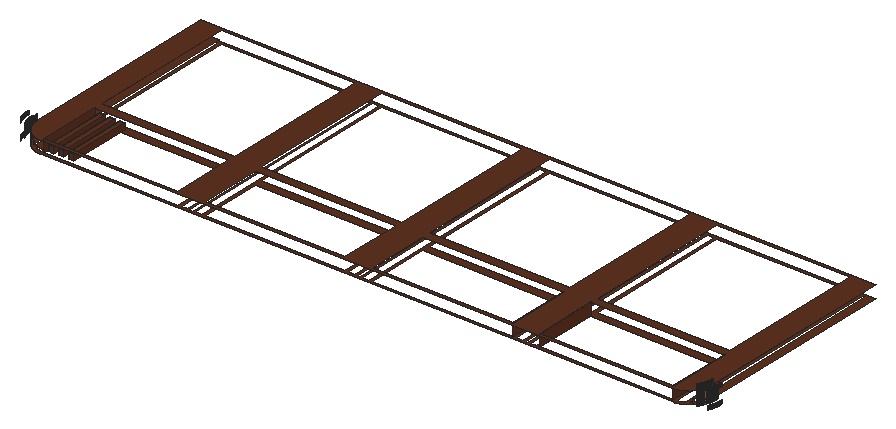
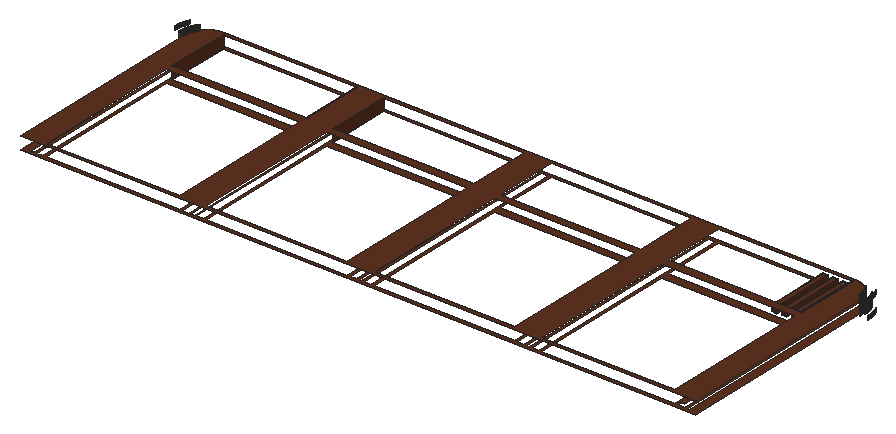
# SketchUp Ruby script. Lengths in inches.
U = 1.inch
M = Sketchup.active_model
def pt(a) = Geom::Point3d.new(a.map { |v| v * U })
def face(e, loops, mat)
  f = e.add_face(loops[0].map { |a| pt(a) })
  loops[1..].each { |l| e.add_face(l.map { |a| pt(a) }).erase! }
  f.material = f.back_material = mat if mat
  f
end
# faces: each face lists its corners as indices into pts; further lists are holes
def faces(e, pts, list, mat = nil) = list.each { |f| face(e, (f[0].is_a?(Array) ? f : [f]).map { |l| l.map { |i| pts[i] } }, mat) }
# xy, xz, yz: faces in a plane at the given z, y or x. An outline is a flat list of corners, or four numbers for a rectangle; further outlines are holes
def ring(l) = l.size == 4 ? [[l[0], l[1]], [l[2], l[1]], [l[2], l[3]], [l[0], l[3]]] : l.each_slice(2).to_a
def flat(e, list, mat, &to3) = list.each { |f| face(e, (f[0].is_a?(Array) ? f : [f]).map { |l| ring(l).map { |u, v| to3.(u, v) } }, mat) }
def xy(e, z, list, mat = nil) = flat(e, list, mat) { |x, y| [x, y, z] }
def xz(e, y, list, mat = nil) = flat(e, list, mat) { |x, z| [x, y, z] }
def yz(e, x, list, mat = nil) = flat(e, list, mat) { |y, z| [x, y, z] }
def lines(e, pts, list) = list.each { |a, b| e.add_line(pt(pts[a]), pt(pts[b])) }
# prism: a flat outline (further loops are holes) pulled along v
def prism(e, loops, v, mat = nil)
  f = face(e, loops, mat); d = Geom::Vector3d.new(v.map { |x| x * U })
  f.pushpull(f.normal.samedirection?(d) ? d.length : -d.length)
end
def box(e, o, s, mat = nil) = prism(e, [[o, [o[0] + s[0], o[1], o[2]], [o[0] + s[0], o[1] + s[1], o[2]], [o[0], o[1] + s[1], o[2]]]], [0, 0, s[2]], mat)
def at(x, y, z, deg = 0) = Geom::Transformation.translation(pt([x, y, z])) * Geom::Transformation.rotation(ORIGIN, Z_AXIS, deg.degrees)
def axes(o, x, y, z) = Geom::Transformation.new([*x, 0, *y, 0, *z, 0, *pt(o).to_a, 1])
def part(name) = M.definitions.add(name)
# library, detail: a bought-in or finely detailed component or shape, given as its bounding box
def library(name, o, s) = part(name).tap { |d| box(d.entities, o, s) }
def detail(e, o, s) = box(e.add_group.entities, o, s)
def put(e, d, t, mat = nil) = e.add_instance(d, t).tap { |i| i.material = mat if mat }
def group(e, t, mat = nil) = e.add_group.tap { |g| g.transformation = t; g.material = mat if mat }.entities
root = M.entities
M.materials.add("1799 AP 8574 BURNISHED CARAMEL").color = [140, 96, 69]
M.materials.add("1816 AP K197 Dark Kaapi-N").color = [79, 50, 27]
M.materials.add("[Wood Cherry Original]1").color = [93, 50, 33]
c1 = part("3")
box(c1.entities,[0,0,0],[3,2,36])
xy(root,391,[[[65.66,83,64.81,83.05,64.13,83.13,63.97,83.16,63.8,83.1875,63.63,83.22,63.46,83.25,63.3,83.28,63.13,83.32,62.97,83.36,62.8,83.4,62.64,83.44,62.47,83.49,62.31,83.54,62.14,83.58,61.98,83.64,61.82,83.69,61.66,83.75,61.5,83.8,61.34,83.86,61.18,83.93,61.03,83.99,60.87,84.06,60.71,84.125,60.56,84.19,60.4,84.27,60.25,84.34,59.65,84.66,59.52,84.73,59.5,84.74,59.35,84.83,59.21,84.92,59.0625,85.01,58.92,85.1,58.78,85.19,58.64,85.29,58.5,85.38,58.22,85.58,58.09,85.6875,57.95,85.79,57.82,85.9,57.6875,86.01,57.56,86.11,57.52,86.15,57.43,86.23,57.3,86.34,57.18,86.45,57.05,86.57,56.93,86.6875,56.81,86.81,56.6875,86.93,56.57,87.05,56.45,87.18,56.34,87.3,56.23,87.43,56.11,87.56,56.01,87.6875,55.9,87.82,55.79,87.95,55.6875,88.09,55.58,88.22,55.38,88.5,55.29,88.64,55.19,88.78,55.1,88.92,55.01,89.0625,54.92,89.21,54.83,89.35,54.74,89.5,54.34,90.25,54.27,90.4,54.19,90.56,54.125,90.71,54.06,90.87,53.99,91.03,53.93,91.18,53.86,91.34,53.8,91.5,53.75,91.66,53.69,91.82,53.64,91.98,53.58,92.14,53.54,92.31,53.49,92.47,53.44,92.64,53.4,92.8,53.36,92.97,53.32,93.13,53.28,93.3,53.25,93.46,53.22,93.63,53.1875,93.8,53.16,93.97,53.13,94.13,53.05,94.81,53,95.66,53,211,433,211,433,95.66,432.95,94.81,432.87,94.13,432.84,93.97,432.8125,93.8,432.78,93.63,432.75,93.46,432.72,93.3,432.68,93.13,432.64,92.97,432.6,92.8,432.56,92.64,432.51,92.47,432.46,92.31,432.42,92.14,432.36,91.98,432.31,91.82,432.25,91.66,432.2,91.5,432.14,91.34,432.07,91.18,432.01,91.03,431.94,90.87,431.875,90.71,431.81,90.56,431.73,90.4,431.66,90.25,431.26,89.5,431.17,89.35,431.08,89.21,430.99,89.0625,430.9,88.92,430.81,88.78,430.71,88.64,430.62,88.5,430.42,88.22,430.3125,88.09,430.21,87.95,430.1,87.82,429.99,87.6875,429.89,87.56,429.77,87.43,429.66,87.3,429.55,87.18,429.43,87.05,429.3125,86.93,429.19,86.81,429.07,86.6875,428.95,86.57,428.82,86.45,428.7,86.34,428.57,86.23,428.48,86.15,428.44,86.11,428.3125,86.01,428.18,85.9,428.05,85.79,427.91,85.6875,427.78,85.58,427.5,85.38,427.36,85.29,427.22,85.19,427.08,85.1,426.9375,85.01,426.79,84.92,426.65,84.83,426.5,84.74,426.48,84.73,426.35,84.66,425.75,84.34,425.6,84.27,425.44,84.19,425.29,84.125,425.13,84.06,424.97,83.99,424.82,83.93,424.66,83.86,424.5,83.8,424.34,83.75,424.18,83.69,424.02,83.64,423.86,83.58,423.69,83.54,423.53,83.49,423.36,83.44,423.2,83.4,423.03,83.36,422.87,83.32,422.7,83.28,422.54,83.25,422.37,83.22,422.2,83.1875,422.03,83.16,421.87,83.13,421.19,83.05,420.34,83],[156.25,124.5,235.5,209.5],[250.5,124.5,329.75,209.5],[66.02,124.5,141.25,209.5],[344.75,124.5,419.98,209.5],[250.5,84.5,329.75,120.5],[156.25,84.5,235.5,120.5],[344.75,84.5,419.98,120.5],[66.02,84.5,141.25,120.5],[142.75,84.5,146.75,209.5],[150.75,84.5,154.75,209.5],[245,84.5,249,209.5],[237,84.5,241,209.5],[339.25,84.5,343.25,209.5],[331.25,84.5,335.25,209.5],[421.48,84.6,421.5,84.6,421.8,84.64,422.1,84.69,422.24,84.72,422.54,84.78,422.83,84.85,423.12,84.93,423.7,85.11,423.98,85.21,424.4,85.375,424.68,85.49,424.95,85.62,425.09,85.6875,425.35,85.82,425.48,85.89,425.48,209.5,421.48,209.5],[64.52,84.61,64.52,209.5,60.52,209.5,60.52,85.9,60.99,85.66,61.47,85.43,61.96,85.24,62.46,85.0625,62.97,84.91,63.48,84.78,64,84.68],[147.75,84.5,149.75,209.5],[242,84.5,244,209.5],[336.25,84.5,338.25,209.5],[426.48,86.5,426.51,86.52,426.64,86.61,427.12,86.97,427.35,87.16,427.47,87.26,427.69,87.45,427.81,87.56,428.02,87.76,428.34,88.08,428.48,88.23,428.48,209.5,426.48,209.5],[59.52,86.5,59.52,209.5,57.52,209.5,57.52,88.23,57.66,88.08,58.08,87.66,58.19,87.56,58.42,87.35,58.88,86.97,59.24,86.7,59.49,86.52]]],"[Wood Cherry Original]1")
xy(root,392.75,[[65.85,84.5,66.02,84.5,65.45,84.52,64.875,84.5625,64.52,84.61,64.3,84.64,63.74,84.74,63.18,84.87,62.625,85.02,62.08,85.2,61.54,85.41,61.02,85.65,60.52,85.9,60.52,209.5,64.52,209.5,64.52,84.6,64.8,84.5625,65.1,84.54,65.55,84.51]],"[Wood Cherry Original]1")
xy(root,398,[[[65.66,83,420.34,83,421.19,83.05,421.87,83.13,422.03,83.16,422.2,83.1875,422.37,83.22,422.54,83.25,422.7,83.28,422.87,83.32,423.03,83.36,423.2,83.4,423.36,83.44,423.53,83.49,423.69,83.54,423.86,83.58,424.02,83.64,424.18,83.69,424.34,83.75,424.5,83.8,424.66,83.86,424.82,83.93,424.97,83.99,425.13,84.06,425.29,84.125,425.44,84.19,425.6,84.27,425.75,84.34,426.5,84.74,426.65,84.83,426.79,84.92,426.9375,85.01,427.08,85.1,427.22,85.19,427.36,85.29,427.5,85.38,427.78,85.58,427.91,85.6875,428.05,85.79,428.18,85.9,428.3125,86.01,428.44,86.11,428.57,86.23,428.7,86.34,428.82,86.45,428.95,86.57,429.07,86.6875,429.19,86.81,429.3125,86.93,429.43,87.05,429.55,87.18,429.66,87.3,429.77,87.43,429.89,87.56,429.99,87.6875,430.1,87.82,430.21,87.95,430.3125,88.09,430.42,88.22,430.62,88.5,430.71,88.64,430.81,88.78,430.9,88.92,430.99,89.0625,431.08,89.21,431.17,89.35,431.26,89.5,431.66,90.25,431.73,90.4,431.81,90.56,431.875,90.71,431.94,90.87,432.01,91.03,432.07,91.18,432.14,91.34,432.2,91.5,432.25,91.66,432.31,91.82,432.36,91.98,432.42,92.14,432.46,92.31,432.51,92.47,432.56,92.64,432.6,92.8,432.64,92.97,432.68,93.13,432.72,93.3,432.75,93.46,432.78,93.63,432.8125,93.8,432.84,93.97,432.87,94.13,432.95,94.81,433,95.66,433,211,53,211,53,95.66,53.05,94.81,53.13,94.13,53.16,93.97,53.1875,93.8,53.22,93.63,53.25,93.46,53.28,93.3,53.32,93.13,53.36,92.97,53.4,92.8,53.44,92.64,53.49,92.47,53.54,92.31,53.58,92.14,53.64,91.98,53.69,91.82,53.75,91.66,53.8,91.5,53.86,91.34,53.93,91.18,53.99,91.03,54.06,90.87,54.125,90.71,54.19,90.56,54.27,90.4,54.34,90.25,54.74,89.5,54.83,89.35,54.92,89.21,55.01,89.0625,55.1,88.92,55.19,88.78,55.29,88.64,55.38,88.5,55.58,88.22,55.6875,88.09,55.79,87.95,55.9,87.82,56.01,87.6875,56.11,87.56,56.23,87.43,56.34,87.3,56.45,87.18,56.57,87.05,56.6875,86.93,56.81,86.81,56.93,86.6875,57.05,86.57,57.18,86.45,57.3,86.34,57.43,86.23,57.56,86.11,57.6875,86.01,57.82,85.9,57.95,85.79,58.09,85.6875,58.22,85.58,58.5,85.38,58.64,85.29,58.78,85.19,58.92,85.1,59.0625,85.01,59.21,84.92,59.35,84.83,59.5,84.74,60.25,84.34,60.4,84.27,60.56,84.19,60.71,84.125,60.87,84.06,61.03,83.99,61.18,83.93,61.34,83.86,61.5,83.8,61.66,83.75,61.82,83.69,61.98,83.64,62.14,83.58,62.31,83.54,62.47,83.49,62.64,83.44,62.8,83.4,62.97,83.36,63.13,83.32,63.3,83.28,63.46,83.25,63.63,83.22,63.8,83.1875,63.97,83.16,64.13,83.13,64.81,83.05],[344.75,84.5,344.75,209.5,419.98,209.5,419.98,124.5,344.75,124.5,344.75,120.5,419.98,120.5,419.98,84.5],[156.25,124.5,235.5,209.5],[250.5,124.5,329.75,209.5],[66.02,124.5,141.25,209.5],[250.5,84.5,329.75,120.5],[156.25,84.5,235.5,120.5],[66.02,84.5,141.25,120.5]]],"[Wood Cherry Original]1")
yz(root,48,[[95.76,390,96,392],[95.76,399,96,401]],"1816 AP K197 Dark Kaapi-N")
yz(root,48.01,[[95.29,390,95.53,392],[95.29,399,95.53,401]],"1816 AP K197 Dark Kaapi-N")
yz(root,50,[[95.79,392,96.01,399]],"1799 AP 8574 BURNISHED CARAMEL")
yz(root,50.01,[[95.37,392,95.58,399]],"1799 AP 8574 BURNISHED CARAMEL")
yz(root,53,[[95.66,390,95.83,401],[95.83,390,96.02,401]],"1816 AP K197 Dark Kaapi-N")
yz(root,53,[[95.66,391,95.83,398],[95.83,391,96.02,398]],"[Wood Cherry Original]1")
yz(root,66.02,[[84.5,391,120.5,398]],"[Wood Cherry Original]1")
yz(root,329.75,[[84.5,391,120.5,398]],"[Wood Cherry Original]1")
yz(root,344.75,[[84.5,391,120.5,398]],"[Wood Cherry Original]1")
yz(root,419.98,[[84.5,391,120.5,398]],"[Wood Cherry Original]1")
yz(root,433,[[95.66,390,95.83,401],[95.83,390,96.02,401]],"1816 AP K197 Dark Kaapi-N")
yz(root,433,[[95.66,391,95.83,398],[95.83,391,96.02,398]],"[Wood Cherry Original]1")
yz(root,435.99,[[95.37,392,95.58,399]],"1799 AP 8574 BURNISHED CARAMEL")
yz(root,436,[[95.79,392,96.01,399]],"1799 AP 8574 BURNISHED CARAMEL")
yz(root,437.99,[[95.29,390,95.53,392],[95.29,399,95.53,401]],"1816 AP K197 Dark Kaapi-N")
yz(root,438,[[95.76,390,96,392],[95.76,399,96,401]],"1816 AP K197 Dark Kaapi-N")
p = [[55.58,88.22,401],[55.6875,88.09,401],[55.6875,88.09,390],[55.58,88.22,390],[430.3125,88.09,401],[430.42,88.22,401],
  [430.42,88.22,390],[430.3125,88.09,390],[55.48,88.36,401],[55.48,88.36,390],[430.52,88.36,401],[430.52,88.36,390],
  [49.65,88.46,390],[49.75,88.25,390],[49.75,88.25,392],[49.65,88.46,392],[436.25,88.25,390],[436.35,88.46,390],
  [436.35,88.46,392],[436.25,88.25,392],[55.38,88.5,401],[55.38,88.5,390],[430.62,88.5,401],[430.62,88.5,390],
  [49.56,88.68,390],[49.56,88.68,392],[55.29,88.64,401],[55.29,88.64,390],[430.71,88.64,401],[430.71,88.64,390],
  [436.44,88.68,390],[436.44,88.68,392],[55.19,88.78,401],[55.19,88.78,390],[430.81,88.78,401],[430.81,88.78,390],
  [49.46,88.89,390],[49.46,88.89,392],[436.54,88.89,390],[436.54,88.89,392],[55.1,88.92,401],[55.1,88.92,390],
  [430.9,88.92,401],[430.9,88.92,390],[49.37,89.11,390],[49.37,89.11,392],[55.01,89.0625,401],[55.01,89.0625,390],
  [430.99,89.0625,401],[430.99,89.0625,390],[436.63,89.11,390],[436.63,89.11,392],[49.28,89.33,390],[49.28,89.33,392],
  [54.92,89.21,401],[54.92,89.21,390],[431.08,89.21,401],[431.08,89.21,390],[436.72,89.33,390],[436.72,89.33,392],
  [54.83,89.35,401],[54.83,89.35,390],[431.17,89.35,401],[431.17,89.35,390],[49.2,89.55,390],[49.2,89.55,392],
  [436.8,89.55,390],[436.8,89.55,392],[54.74,89.5,401],[54.74,89.5,390],[431.26,89.5,401],[431.26,89.5,390],
  [49.11,89.77,390],[49.11,89.77,392],[54.66,89.65,401],[54.66,89.65,390],[431.34,89.65,401],[431.34,89.65,390],
  [436.89,89.77,390],[436.89,89.77,392],[54.58,89.8,401],[54.58,89.8,390],[431.42,89.8,401],[431.42,89.8,390],
  [49.03,89.99,390],[49.03,89.99,392],[54.5,89.95,401],[54.5,89.95,390],[431.5,89.95,401],[431.5,89.95,390],
  [436.97,89.99,390],[436.97,89.99,392],[54.42,90.1,401],[54.42,90.1,390],[431.58,90.1,401],[431.58,90.1,390],
  [48.96,90.21,390],[48.96,90.21,392],[437.04,90.21,390],[437.04,90.21,392],[54.34,90.25,401],[54.34,90.25,390],
  [431.66,90.25,401],[431.66,90.25,390],[48.88,90.4375,390],[48.88,90.4375,392],[437.12,90.4375,390],[437.12,90.4375,392],
  [54.27,90.4,401],[54.27,90.4,390],[431.73,90.4,401],[431.73,90.4,390],[48.81,90.66,390],[48.81,90.66,392],
  [54.19,90.56,401],[54.19,90.56,390],[431.81,90.56,401],[431.81,90.56,390],[437.19,90.66,390],[437.19,90.66,392],
  [54.125,90.71,401],[54.125,90.71,390],[431.875,90.71,401],[431.875,90.71,390],[48.74,90.89,390],[48.74,90.89,392],
  [54.06,90.87,401],[54.06,90.87,390],[431.94,90.87,401],[431.94,90.87,390],[437.26,90.89,390],[437.26,90.89,392],
  [48.68,91.11,390],[48.68,91.11,392],[53.99,91.03,401],[53.99,91.03,390],[432.01,91.03,401],[432.01,91.03,390],
  [437.32,91.11,390],[437.32,91.11,392],[53.93,91.18,401],[53.93,91.18,390],[432.07,91.18,401],[432.07,91.18,390],
  [48.61,91.34,390],[48.61,91.34,392],[437.39,91.34,390],[437.39,91.34,392],[53.86,91.34,401],[53.86,91.34,390],
  [432.14,91.34,401],[432.14,91.34,390],[48.55,91.57,390],[48.55,91.57,392],[53.8,91.5,401],[53.8,91.5,390],
  [432.2,91.5,401],[432.2,91.5,390],[437.45,91.57,390],[437.45,91.57,392],[53.75,91.66,401],[53.75,91.66,390],
  [432.25,91.66,401],[432.25,91.66,390],[48.5,91.8,390],[48.5,91.8,392],[437.5,91.8,390],[437.5,91.8,392],
  [53.69,91.82,401],[53.69,91.82,390],[432.31,91.82,401],[432.31,91.82,390],[48.44,92.03,390],[48.44,92.03,392],
  [53.64,91.98,401],[53.64,91.98,390],[432.36,91.98,401],[432.36,91.98,390],[437.56,92.03,390],[437.56,92.03,392],
  [48.39,92.26,390],[48.39,92.26,392],[53.58,92.14,401],[53.58,92.14,390],[432.42,92.14,401],[432.42,92.14,390],
  [437.61,92.26,390],[437.61,92.26,392],[53.54,92.31,401],[53.54,92.31,390],[432.46,92.31,401],[432.46,92.31,390],
  [48.35,92.49,390],[48.35,92.49,392],[53.49,92.47,401],[53.49,92.47,390],[432.51,92.47,401],[432.51,92.47,390],
  [437.65,92.49,390],[437.65,92.49,392],[48.3,92.72,390],[48.3,92.72,392],[53.44,92.64,401],[53.44,92.64,390],
  [432.56,92.64,401],[432.56,92.64,390],[437.7,92.72,390],[437.7,92.72,392],[53.4,92.8,401],[53.4,92.8,390],
  [432.6,92.8,401],[432.6,92.8,390],[48.26,92.95,390],[48.26,92.95,392],[437.74,92.95,390],[437.74,92.95,392],
  [53.36,92.97,401],[53.36,92.97,390],[432.64,92.97,401],[432.64,92.97,390],[48.22,93.18,390],[48.22,93.18,392],
  [53.32,93.13,401],[53.32,93.13,390],[432.68,93.13,401],[432.68,93.13,390],[437.78,93.18,390],[437.78,93.18,392],
  [53.28,93.3,401],[53.28,93.3,390],[432.72,93.3,401],[432.72,93.3,390],[48.1875,93.42,390],[48.1875,93.42,392],
  [437.8125,93.42,390],[437.8125,93.42,392],[53.25,93.46,401],[53.25,93.46,390],[432.75,93.46,401],[432.75,93.46,390],
  [48.15,93.65,390],[48.15,93.65,392],[437.85,93.65,390],[437.85,93.65,392],[53.22,93.63,401],[53.22,93.63,390],
  [432.78,93.63,401],[432.78,93.63,390],[53.1875,93.8,401],[53.1875,93.8,390],[432.8125,93.8,401],[432.8125,93.8,390],
  [48.125,93.88,390],[48.125,93.88,392],[437.875,93.88,390],[437.875,93.88,392],[53.16,93.97,401],[53.16,93.97,390],
  [432.84,93.97,401],[432.84,93.97,390],[48.1,94.12,390],[48.1,94.12,392],[437.9,94.12,390],[437.9,94.12,392],
  [53.13,94.13,401],[53.13,94.13,390],[432.87,94.13,401],[432.87,94.13,390],[48.08,94.35,390],[48.08,94.35,392],
  [53.11,94.3,401],[53.11,94.3,390],[432.89,94.3,401],[432.89,94.3,390],[437.92,94.35,390],[437.92,94.35,392],
  [53.09,94.47,401],[53.09,94.47,390],[432.91,94.47,401],[432.91,94.47,390],[48.06,94.59,390],[48.06,94.59,392],
  [437.94,94.59,390],[437.94,94.59,392],[53.07,94.64,401],[53.07,94.64,390],[432.93,94.64,401],[432.93,94.64,390],
  [48.04,94.82,390],[48.04,94.82,392],[53.05,94.81,401],[53.05,94.81,390],[432.95,94.81,401],[432.95,94.81,390],
  [437.96,94.82,390],[437.96,94.82,392],[48.02,95.06,390],[48.02,95.06,392],[53.04,94.98,401],[53.04,94.98,390],
  [432.96,94.98,401],[432.96,94.98,390],[437.98,95.06,390],[437.98,95.06,392],[53.03,95.15,401],[53.03,95.15,390],
  [432.97,95.15,401],[432.97,95.15,390],[48.01,95.29,390],[48.01,95.29,392],[53.02,95.32,401],[53.02,95.32,390],
  [432.98,95.32,401],[432.98,95.32,390],[437.99,95.29,390],[437.99,95.29,392],[53.01,95.49,401],[53.01,95.49,390],
  [432.99,95.49,401],[432.99,95.49,390],[48,95.76,390],[48.01,95.53,390],[48.01,95.53,392],[48,95.76,392],
  [53,95.66,401],[53,95.66,390],[433,95.66,401],[433,95.66,390],[437.99,95.53,390],[438,95.76,390],
  [438,95.76,392],[437.99,95.53,392],[55.58,88.22,391],[55.6875,88.09,391],[55.6875,88.09,398],[55.58,88.22,398],
  [57.66,88.08,391],[57.52,88.23,391],[57.52,88.23,392.75],[57.66,88.08,392.75],[428.48,88.23,391],[428.34,88.08,391],
  [428.34,88.08,392.75],[428.48,88.23,392.75],[430.3125,88.09,391],[430.42,88.22,391],[430.42,88.22,398],[430.3125,88.09,398],
  [55.48,88.36,391],[55.48,88.36,398],[430.52,88.36,391],[430.52,88.36,398],[55.38,88.5,391],[55.38,88.5,398],
  [430.62,88.5,391],[430.62,88.5,398],[55.29,88.64,391],[55.29,88.64,398],[430.71,88.64,391],[430.71,88.64,398],
  [55.19,88.78,391],[55.19,88.78,398],[430.81,88.78,391],[430.81,88.78,398],[55.1,88.92,391],[55.1,88.92,398],
  [430.9,88.92,391],[430.9,88.92,398],[55.01,89.0625,391],[55.01,89.0625,398],[430.99,89.0625,391],[430.99,89.0625,398],
  [54.92,89.21,391],[54.92,89.21,398],[431.08,89.21,391],[431.08,89.21,398],[54.83,89.35,391],[54.83,89.35,398],
  [431.17,89.35,391],[431.17,89.35,398],[54.74,89.5,391],[54.74,89.5,398],[431.26,89.5,391],[431.26,89.5,398],
  [54.66,89.65,391],[54.66,89.65,398],[431.34,89.65,391],[431.34,89.65,398],[54.58,89.8,391],[54.58,89.8,398],
  [431.42,89.8,391],[431.42,89.8,398],[54.5,89.95,391],[54.5,89.95,398],[431.5,89.95,391],[431.5,89.95,398],
  [54.42,90.1,391],[54.42,90.1,398],[431.58,90.1,391],[431.58,90.1,398],[54.34,90.25,391],[54.34,90.25,398],
  [431.66,90.25,391],[431.66,90.25,398],[54.27,90.4,391],[54.27,90.4,398],[431.73,90.4,391],[431.73,90.4,398],
  [54.19,90.56,391],[54.19,90.56,398],[431.81,90.56,391],[431.81,90.56,398],[54.125,90.71,391],[54.125,90.71,398],
  [431.875,90.71,391],[431.875,90.71,398],[54.06,90.87,391],[54.06,90.87,398],[431.94,90.87,391],[431.94,90.87,398],
  [53.99,91.03,391],[53.99,91.03,398],[432.01,91.03,391],[432.01,91.03,398],[53.93,91.18,391],[53.93,91.18,398],
  [432.07,91.18,391],[432.07,91.18,398],[53.86,91.34,391],[53.86,91.34,398],[432.14,91.34,391],[432.14,91.34,398],
  [53.8,91.5,391],[53.8,91.5,398],[432.2,91.5,391],[432.2,91.5,398],[53.75,91.66,391],[53.75,91.66,398],
  [432.25,91.66,391],[432.25,91.66,398],[53.69,91.82,391],[53.69,91.82,398],[432.31,91.82,391],[432.31,91.82,398],
  [53.64,91.98,391],[53.64,91.98,398],[432.36,91.98,391],[432.36,91.98,398],[53.58,92.14,391],[53.58,92.14,398],
  [432.42,92.14,391],[432.42,92.14,398],[53.54,92.31,391],[53.54,92.31,398],[432.46,92.31,391],[432.46,92.31,398],
  [53.49,92.47,391],[53.49,92.47,398],[432.51,92.47,391],[432.51,92.47,398],[53.44,92.64,391],[53.44,92.64,398],
  [432.56,92.64,391],[432.56,92.64,398],[53.4,92.8,391],[53.4,92.8,398],[432.6,92.8,391],[432.6,92.8,398],
  [53.36,92.97,391],[53.36,92.97,398],[432.64,92.97,391],[432.64,92.97,398],[53.32,93.13,391],[53.32,93.13,398],
  [432.68,93.13,391],[432.68,93.13,398],[53.28,93.3,391],[53.28,93.3,398],[432.72,93.3,391],[432.72,93.3,398],
  [53.25,93.46,391],[53.25,93.46,398],[432.75,93.46,391],[432.75,93.46,398],[53.22,93.63,391],[53.22,93.63,398],
  [432.78,93.63,391],[432.78,93.63,398],[53.1875,93.8,391],[53.1875,93.8,398],[432.8125,93.8,391],[432.8125,93.8,398],
  [53.16,93.97,391],[53.16,93.97,398],[432.84,93.97,391],[432.84,93.97,398],[53.13,94.13,391],[53.13,94.13,398],
  [432.87,94.13,391],[432.87,94.13,398],[53.11,94.3,391],[53.11,94.3,398],[432.89,94.3,391],[432.89,94.3,398],
  [53.09,94.47,391],[53.09,94.47,398],[432.91,94.47,391],[432.91,94.47,398],[53.07,94.64,391],[53.07,94.64,398],
  [432.93,94.64,391],[432.93,94.64,398],[53.05,94.81,391],[53.05,94.81,398],[432.95,94.81,391],[432.95,94.81,398],
  [53.04,94.98,391],[53.04,94.98,398],[432.96,94.98,391],[432.96,94.98,398],[53.03,95.15,391],[53.03,95.15,398],
  [432.97,95.15,391],[432.97,95.15,398],[53.02,95.32,391],[53.02,95.32,398],[432.98,95.32,391],[432.98,95.32,398],
  [53.01,95.49,391],[53.01,95.49,398],[432.99,95.49,391],[432.99,95.49,398],[53,95.66,391],[53,95.66,398],
  [433,95.66,391],[433,95.66,398],[51.9375,88.37,392],[52.04,88.18,392],[52.04,88.18,399],[51.9375,88.37,399],
  [433.96,88.18,392],[434.0625,88.37,392],[434.0625,88.37,399],[433.96,88.18,399],[51.84,88.55,392],[51.84,88.55,399],
  [434.16,88.55,392],[434.16,88.55,399],[51.74,88.74,392],[51.74,88.74,399],[434.26,88.74,392],[434.26,88.74,399],
  [51.65,88.92,392],[51.65,88.92,399],[434.35,88.92,392],[434.35,88.92,399],[51.56,89.11,392],[51.56,89.11,399],
  [434.44,89.11,392],[434.44,89.11,399],[51.47,89.3,392],[51.47,89.3,399],[434.53,89.3,392],[434.53,89.3,399],
  [51.38,89.49,392],[51.38,89.49,399],[434.62,89.49,392],[434.62,89.49,399],[51.3,89.68,392],[51.3,89.68,399],
  [434.7,89.68,392],[434.7,89.68,399],[51.22,89.88,392],[51.22,89.88,399],[434.78,89.88,392],[434.78,89.88,399],
  [51.14,90.07,392],[51.14,90.07,399],[434.86,90.07,392],[434.86,90.07,399],[51.0625,90.27,392],[51.0625,90.27,399],
  [434.9375,90.27,392],[434.9375,90.27,399],[50.99,90.46,392],[50.99,90.46,399],[435.01,90.46,392],[435.01,90.46,399],
  [50.92,90.66,392],[50.92,90.66,399],[435.08,90.66,392],[435.08,90.66,399],[50.85,90.86,392],[50.85,90.86,399],
  [435.15,90.86,392],[435.15,90.86,399],[50.78,91.06,392],[50.78,91.06,399],[435.22,91.06,392],[435.22,91.06,399],
  [50.72,91.26,392],[50.72,91.26,399],[435.28,91.26,392],[435.28,91.26,399],[50.66,91.46,392],[50.66,91.46,399],
  [435.34,91.46,392],[435.34,91.46,399],[50.6,91.66,392],[50.6,91.66,399],[435.4,91.66,392],[435.4,91.66,399],
  [50.55,91.86,392],[50.55,91.86,399],[435.45,91.86,392],[435.45,91.86,399],[50.49,92.0625,392],[50.49,92.0625,399],
  [435.51,92.0625,392],[435.51,92.0625,399],[50.44,92.26,392],[50.44,92.26,399],[435.56,92.26,392],[435.56,92.26,399],
  [50.39,92.47,392],[50.39,92.47,399],[435.61,92.47,392],[435.61,92.47,399],[50.35,92.67,392],[50.35,92.67,399],
  [435.65,92.67,392],[435.65,92.67,399],[50.31,92.88,392],[50.31,92.88,399],[435.69,92.88,392],[435.69,92.88,399],
  [50.27,93.08,392],[50.27,93.08,399],[435.73,93.08,392],[435.73,93.08,399],[50.23,93.29,392],[50.23,93.29,399],
  [435.77,93.29,392],[435.77,93.29,399],[50.2,93.5,392],[50.2,93.5,399],[435.8,93.5,392],[435.8,93.5,399],
  [50.17,93.7,392],[50.17,93.7,399],[435.83,93.7,392],[435.83,93.7,399],[50.14,93.91,392],[50.14,93.91,399],
  [435.86,93.91,392],[435.86,93.91,399],[50.11,94.12,392],[50.11,94.12,399],[435.89,94.12,392],[435.89,94.12,399],
  [50.09,94.33,392],[50.09,94.33,399],[435.91,94.33,392],[435.91,94.33,399],[50.07,94.54,392],[50.07,94.54,399],
  [435.93,94.54,392],[435.93,94.54,399],[50.05,94.74,392],[50.05,94.74,399],[435.95,94.74,392],[435.95,94.74,399],
  [50.03,94.95,392],[50.03,94.95,399],[435.97,94.95,392],[435.97,94.95,399],[50.02,95.16,392],[50.02,95.16,399],
  [435.98,95.16,392],[435.98,95.16,399],[50.01,95.37,392],[50.01,95.37,399],[435.99,95.37,392],[435.99,95.37,399],
  [50,95.79,392],[50.01,95.58,392],[50.01,95.58,399],[50,95.79,399],[435.99,95.58,392],[436,95.79,392],
  [436,95.79,399],[435.99,95.58,399],[49.75,88.25,399],[49.86,88.04,399],[49.86,88.04,401],[49.75,88.25,401],
  [436.14,88.04,399],[436.25,88.25,399],[436.25,88.25,401],[436.14,88.04,401],[49.65,88.46,399],[49.65,88.46,401],
  [436.35,88.46,399],[436.35,88.46,401],[49.56,88.68,399],[49.56,88.68,401],[436.44,88.68,399],[436.44,88.68,401],
  [49.46,88.89,399],[49.46,88.89,401],[436.54,88.89,399],[436.54,88.89,401],[49.37,89.11,399],[49.37,89.11,401],
  [436.63,89.11,399],[436.63,89.11,401],[49.28,89.33,399],[49.28,89.33,401],[436.72,89.33,399],[436.72,89.33,401],
  [49.2,89.55,399],[49.2,89.55,401],[436.8,89.55,399],[436.8,89.55,401],[49.11,89.77,399],[49.11,89.77,401],
  [436.89,89.77,399],[436.89,89.77,401],[49.03,89.99,399],[49.03,89.99,401],[436.97,89.99,399],[436.97,89.99,401],
  [48.96,90.21,399],[48.96,90.21,401],[437.04,90.21,399],[437.04,90.21,401],[48.88,90.4375,399],[48.88,90.4375,401],
  [437.12,90.4375,399],[437.12,90.4375,401],[48.81,90.66,399],[48.81,90.66,401],[437.19,90.66,399],[437.19,90.66,401],
  [48.74,90.89,399],[48.74,90.89,401],[437.26,90.89,399],[437.26,90.89,401],[48.68,91.11,399],[48.68,91.11,401],
  [437.32,91.11,399],[437.32,91.11,401],[48.61,91.34,399],[48.61,91.34,401],[437.39,91.34,399],[437.39,91.34,401],
  [48.55,91.57,399],[48.55,91.57,401],[437.45,91.57,399],[437.45,91.57,401],[48.5,91.8,399],[48.5,91.8,401],
  [437.5,91.8,399],[437.5,91.8,401],[48.44,92.03,399],[48.44,92.03,401],[437.56,92.03,399],[437.56,92.03,401],
  [48.39,92.26,399],[48.39,92.26,401],[437.61,92.26,399],[437.61,92.26,401],[48.35,92.49,399],[48.35,92.49,401],
  [437.65,92.49,399],[437.65,92.49,401],[48.3,92.72,399],[48.3,92.72,401],[437.7,92.72,399],[437.7,92.72,401],
  [48.26,92.95,399],[48.26,92.95,401],[437.74,92.95,399],[437.74,92.95,401],[48.22,93.18,399],[48.22,93.18,401],
  [437.78,93.18,399],[437.78,93.18,401],[48.1875,93.42,399],[48.1875,93.42,401],[437.8125,93.42,399],[437.8125,93.42,401],
  [48.15,93.65,399],[48.15,93.65,401],[437.85,93.65,399],[437.85,93.65,401],[48.125,93.88,399],[48.125,93.88,401],
  [437.875,93.88,399],[437.875,93.88,401],[48.1,94.12,399],[48.1,94.12,401],[437.9,94.12,399],[437.9,94.12,401],
  [48.08,94.35,399],[48.08,94.35,401],[437.92,94.35,399],[437.92,94.35,401],[48.06,94.59,399],[48.06,94.59,401],
  [437.94,94.59,399],[437.94,94.59,401],[48.04,94.82,399],[48.04,94.82,401],[437.96,94.82,399],[437.96,94.82,401],
  [48.02,95.06,399],[48.02,95.06,401],[437.98,95.06,399],[437.98,95.06,401],[48.01,95.29,399],[48.01,95.29,401],
  [437.99,95.29,399],[437.99,95.29,401],[48,95.76,399],[48.01,95.53,399],[48.01,95.53,401],[48,95.76,401],
  [437.99,95.53,399],[438,95.76,399],[438,95.76,401],[437.99,95.53,401]]
faces(root,p,[[0,1,2,3],[4,5,6,7],[8,0,3,9],[5,10,11,6],[12,13,14,15],[16,17,18,19],[20,8,9,21],[10,22,23,11],
  [24,12,15,25],[26,20,21,27],[22,28,29,23],[17,30,31,18],[32,26,27,33],[28,34,35,29],[36,24,25,37],[30,38,39,31],
  [40,32,33,41],[34,42,43,35],[44,36,37,45],[46,40,41,47],[42,48,49,43],[38,50,51,39],[52,44,45,53],[54,46,47,55],
  [48,56,57,49],[50,58,59,51],[60,54,55,61],[56,62,63,57],[64,52,53,65],[58,66,67,59],[68,60,61,69],[62,70,71,63],
  [72,64,65,73],[74,68,69,75],[70,76,77,71],[66,78,79,67],[80,74,75,81],[76,82,83,77],[84,72,73,85],[86,80,81,87],
  [82,88,89,83],[78,90,91,79],[92,86,87,93],[88,94,95,89],[96,84,85,97],[90,98,99,91],[100,92,93,101],[94,102,103,95],
  [104,96,97,105],[98,106,107,99],[108,100,101,109],[102,110,111,103],[112,104,105,113],[114,108,109,115],[110,116,117,111],[106,118,119,107],
  [120,114,115,121],[116,122,123,117],[124,112,113,125],[126,120,121,127],[122,128,129,123],[118,130,131,119],[132,124,125,133],[134,126,127,135],
  [128,136,137,129],[130,138,139,131],[140,134,135,141],[136,142,143,137],[144,132,133,145],[138,146,147,139],[148,140,141,149],[142,150,151,143],
  [152,144,145,153],[154,148,149,155],[150,156,157,151],[146,158,159,147],[160,154,155,161],[156,162,163,157],[164,152,153,165],[158,166,167,159],
  [168,160,161,169],[162,170,171,163],[172,164,165,173],[174,168,169,175],[170,176,177,171],[166,178,179,167],[180,172,173,181],[182,174,175,183],
  [176,184,185,177],[178,186,187,179],[188,182,183,189],[184,190,191,185],[192,180,181,193],[194,188,189,195],[190,196,197,191],[186,198,199,187],
  [200,192,193,201],[202,194,195,203],[196,204,205,197],[198,206,207,199],[208,202,203,209],[204,210,211,205],[212,200,201,213],[206,214,215,207],
  [216,208,209,217],[210,218,219,211],[220,212,213,221],[222,216,217,223],[218,224,225,219],[214,226,227,215],[228,222,223,229],[224,230,231,225],
  [232,220,221,233],[226,234,235,227],[236,228,229,237],[230,238,239,231],[240,232,233,241],[234,242,243,235],[244,236,237,245],[238,246,247,239],
  [248,244,245,249],[246,250,251,247],[252,240,241,253],[242,254,255,243],[256,248,249,257],[250,258,259,251],[260,252,253,261],[254,262,263,255],
  [264,256,257,265],[258,266,267,259],[268,260,261,269],[270,264,265,271],[266,272,273,267],[262,274,275,263],[276,270,271,277],[272,278,279,273],
  [280,268,269,281],[274,282,283,275],[284,276,277,285],[278,286,287,279],[288,280,281,289],[290,284,285,291],[286,292,293,287],[282,294,295,283],
  [296,288,289,297],[298,290,291,299],[292,300,301,293],[294,302,303,295],[304,298,299,305],[300,306,307,301],[308,296,297,309],[310,304,305,311],
  [306,312,313,307],[302,314,315,303],[316,310,311,317],[312,318,319,313],[320,321,322,323],[324,316,317,325],[318,326,327,319],[328,329,330,331],
  [692,693,694,695],[696,697,698,699],[700,692,695,701],[697,702,703,698],[704,700,701,705],[702,706,707,703],[708,704,705,709],[706,710,711,707],
  [712,708,709,713],[710,714,715,711],[716,712,713,717],[714,718,719,715],[720,716,717,721],[718,722,723,719],[724,720,721,725],[722,726,727,723],
  [728,724,725,729],[726,730,731,727],[732,728,729,733],[730,734,735,731],[736,732,733,737],[734,738,739,735],[740,736,737,741],[738,742,743,739],
  [744,740,741,745],[742,746,747,743],[748,744,745,749],[746,750,751,747],[752,748,749,753],[750,754,755,751],[756,752,753,757],[754,758,759,755],
  [760,756,757,761],[758,762,763,759],[764,760,761,765],[762,766,767,763],[768,764,765,769],[766,770,771,767],[772,768,769,773],[770,774,775,771],
  [776,772,773,777],[774,778,779,775],[780,776,777,781],[778,782,783,779],[784,780,781,785],[782,786,787,783],[788,784,785,789],[786,790,791,787],
  [792,788,789,793],[790,794,795,791],[796,792,793,797],[794,798,799,795],[800,796,797,801],[798,802,803,799],[804,800,801,805],[802,806,807,803],
  [808,804,805,809],[806,810,811,807],[812,808,809,813],[810,814,815,811],[816,812,813,817],[814,818,819,815],[820,816,817,821],[818,822,823,819],
  [824,825,826,827],[828,829,830,831]],"1816 AP K197 Dark Kaapi-N")
faces(root,p,[[332,333,334,335],[336,337,338,339],[340,341,342,343],[344,345,346,347],[348,332,335,349],[345,350,351,346],[352,348,349,353],[350,354,355,351],
  [356,352,353,357],[354,358,359,355],[360,356,357,361],[358,362,363,359],[364,360,361,365],[362,366,367,363],[368,364,365,369],[366,370,371,367],
  [372,368,369,373],[370,374,375,371],[376,372,373,377],[374,378,379,375],[380,376,377,381],[378,382,383,379],[384,380,381,385],[382,386,387,383],
  [388,384,385,389],[386,390,391,387],[392,388,389,393],[390,394,395,391],[396,392,393,397],[394,398,399,395],[400,396,397,401],[398,402,403,399],
  [404,400,401,405],[402,406,407,403],[408,404,405,409],[406,410,411,407],[412,408,409,413],[410,414,415,411],[416,412,413,417],[414,418,419,415],
  [420,416,417,421],[418,422,423,419],[424,420,421,425],[422,426,427,423],[428,424,425,429],[426,430,431,427],[432,428,429,433],[430,434,435,431],
  [436,432,433,437],[434,438,439,435],[440,436,437,441],[438,442,443,439],[444,440,441,445],[442,446,447,443],[448,444,445,449],[446,450,451,447],
  [452,448,449,453],[450,454,455,451],[456,452,453,457],[454,458,459,455],[460,456,457,461],[458,462,463,459],[464,460,461,465],[462,466,467,463],
  [468,464,465,469],[466,470,471,467],[472,468,469,473],[470,474,475,471],[476,472,473,477],[474,478,479,475],[480,476,477,481],[478,482,483,479],
  [484,480,481,485],[482,486,487,483],[488,484,485,489],[486,490,491,487],[492,488,489,493],[490,494,495,491],[496,492,493,497],[494,498,499,495],
  [500,496,497,501],[498,502,503,499],[504,500,501,505],[502,506,507,503],[508,504,505,509],[506,510,511,507],[512,508,509,513],[510,514,515,511],
  [516,512,513,517],[514,518,519,515],[520,516,517,521],[518,522,523,519],[524,520,521,525],[522,526,527,523],[528,524,525,529],[526,530,531,527],
  [532,528,529,533],[530,534,535,531]],"[Wood Cherry Original]1")
faces(root,p,[[536,537,538,539],[540,541,542,543],[544,536,539,545],[541,546,547,542],[548,544,545,549],[546,550,551,547],[552,548,549,553],[550,554,555,551],
  [556,552,553,557],[554,558,559,555],[560,556,557,561],[558,562,563,559],[564,560,561,565],[562,566,567,563],[568,564,565,569],[566,570,571,567],
  [572,568,569,573],[570,574,575,571],[576,572,573,577],[574,578,579,575],[580,576,577,581],[578,582,583,579],[584,580,581,585],[582,586,587,583],
  [588,584,585,589],[586,590,591,587],[592,588,589,593],[590,594,595,591],[596,592,593,597],[594,598,599,595],[600,596,597,601],[598,602,603,599],
  [604,600,601,605],[602,606,607,603],[608,604,605,609],[606,610,611,607],[612,608,609,613],[610,614,615,611],[616,612,613,617],[614,618,619,615],
  [620,616,617,621],[618,622,623,619],[624,620,621,625],[622,626,627,623],[628,624,625,629],[626,630,631,627],[632,628,629,633],[630,634,635,631],
  [636,632,633,637],[634,638,639,635],[640,636,637,641],[638,642,643,639],[644,640,641,645],[642,646,647,643],[648,644,645,649],[646,650,651,647],
  [652,648,649,653],[650,654,655,651],[656,652,653,657],[654,658,659,655],[660,656,657,661],[658,662,663,659],[664,660,661,665],[662,666,667,663],
  [668,664,665,669],[666,670,671,667],[672,668,669,673],[670,674,675,671],[676,672,673,677],[674,678,679,675],[680,676,677,681],[678,682,683,679],
  [684,685,686,687],[688,689,690,691]],"1799 AP 8574 BURNISHED CARAMEL")
put(root,c1,axes([68.52,120.5,392.75],[1,0,0],[0,0,1.75],[0,-1,0]),"[Wood Cherry Original]1")
put(root,c1,axes([74.125,120.5,392.75],[1,0,0],[0,0,1.75],[0,-1,0]),"[Wood Cherry Original]1")
put(root,c1,axes([79.73,120.5,392.75],[1,0,0],[0,0,1.75],[0,-1,0]),"[Wood Cherry Original]1")
